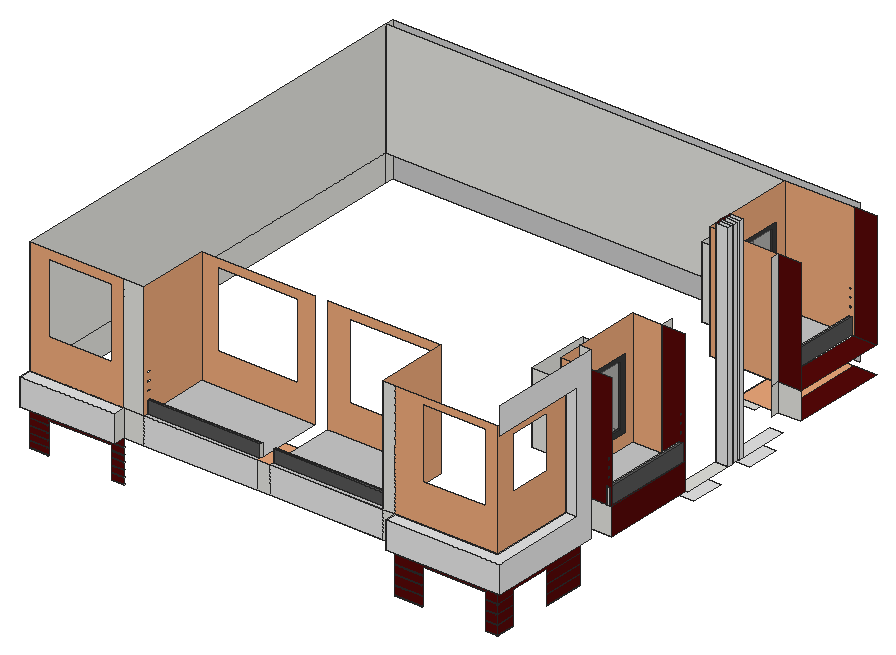
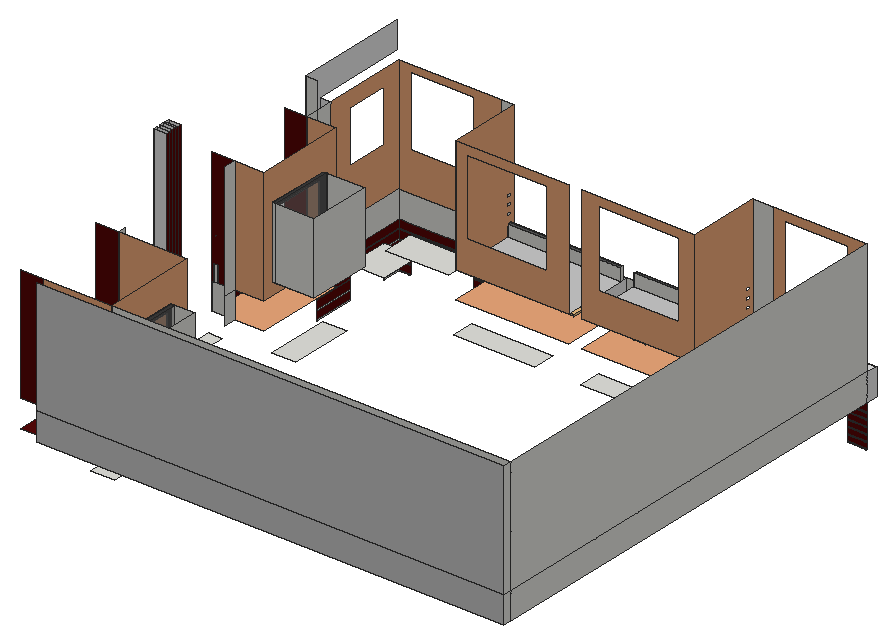
# SketchUp Ruby script. Lengths in inches.
U = 1.inch
M = Sketchup.active_model
def pt(a) = Geom::Point3d.new(a.map { |v| v * U })
def face(e, loops, mat)
  f = e.add_face(loops[0].map { |a| pt(a) })
  loops[1..].each { |l| e.add_face(l.map { |a| pt(a) }).erase! }
  f.material = f.back_material = mat if mat
  f
end
# faces: each face lists its corners as indices into pts; further lists are holes
def faces(e, pts, list, mat = nil) = list.each { |f| face(e, (f[0].is_a?(Array) ? f : [f]).map { |l| l.map { |i| pts[i] } }, mat) }
# xy, xz, yz: faces in a plane at the given z, y or x. An outline is a flat list of corners, or four numbers for a rectangle; further outlines are holes
def ring(l) = l.size == 4 ? [[l[0], l[1]], [l[2], l[1]], [l[2], l[3]], [l[0], l[3]]] : l.each_slice(2).to_a
def flat(e, list, mat, &to3) = list.each { |f| face(e, (f[0].is_a?(Array) ? f : [f]).map { |l| ring(l).map { |u, v| to3.(u, v) } }, mat) }
def xy(e, z, list, mat = nil) = flat(e, list, mat) { |x, y| [x, y, z] }
def xz(e, y, list, mat = nil) = flat(e, list, mat) { |x, z| [x, y, z] }
def yz(e, x, list, mat = nil) = flat(e, list, mat) { |y, z| [x, y, z] }
def lines(e, pts, list) = list.each { |a, b| e.add_line(pt(pts[a]), pt(pts[b])) }
# prism: a flat outline (further loops are holes) pulled along v
def prism(e, loops, v, mat = nil)
  f = face(e, loops, mat); d = Geom::Vector3d.new(v.map { |x| x * U })
  f.pushpull(f.normal.samedirection?(d) ? d.length : -d.length)
end
def box(e, o, s, mat = nil) = prism(e, [[o, [o[0] + s[0], o[1], o[2]], [o[0] + s[0], o[1] + s[1], o[2]], [o[0], o[1] + s[1], o[2]]]], [0, 0, s[2]], mat)
def at(x, y, z, deg = 0) = Geom::Transformation.translation(pt([x, y, z])) * Geom::Transformation.rotation(ORIGIN, Z_AXIS, deg.degrees)
def axes(o, x, y, z) = Geom::Transformation.new([*x, 0, *y, 0, *z, 0, *pt(o).to_a, 1])
def part(name) = M.definitions.add(name)
# library, detail: a bought-in or finely detailed component or shape, given as its bounding box
def library(name, o, s) = part(name).tap { |d| box(d.entities, o, s) }
def detail(e, o, s) = box(e.add_group.entities, o, s)
def put(e, d, t, mat = nil) = e.add_instance(d, t).tap { |i| i.material = mat if mat }
def group(e, t, mat = nil) = e.add_group.tap { |g| g.transformation = t; g.material = mat if mat }.entities
root = M.entities
M.materials.add("Generic").color = [86, 8, 8]
M.materials.add("Generic\#1").color = [236, 168, 122]
M.materials.add("Generic\#4").color = [201, 201, 201]
M.materials.add("Generic\#5").color = [230, 230, 230]
M.materials.add("[Color M06]").color = [86, 86, 86]
M.materials.add("[Color M07]").color = [58, 58, 58]
M.materials.add("[Translucent Glass Gray]").color = [127, 127, 127]
M.materials["[Translucent Glass Gray]"].alpha = 0.35
c1 = library("Tlon Light 450 Ceiling 152 006",[-8.86,-8.86,-3.78],[17.72,17.72,3.56])
c2 = part("Group\#5")
xy(c2.entities,0,[[0,0,6,92.0625]],"[Color M07]")
xy(c2.entities,6.58,[[3,6.58,6,85.48]],"[Color M07]")
xy(c2.entities,96.73,[[3,6.58,6,85.48]],"[Color M07]")
xy(c2.entities,103.3125,[[0,0,6,92.0625]],"[Color M07]")
xz(c2.entities,0,[[0,0,6,103.3125]],"[Color M07]")
xz(c2.entities,6.58,[[3,6.58,6,96.73]],"[Color M07]")
xz(c2.entities,85.48,[[3,6.58,6,96.73]],"[Color M07]")
xz(c2.entities,92.0625,[[0,0,6,103.3125]],"[Color M07]")
yz(c2.entities,0,[[0,0,92.0625,103.3125]],"[Translucent Glass Gray]")
yz(c2.entities,3,[[6.58,6.58,85.48,96.73]],"[Translucent Glass Gray]")
yz(c2.entities,6,[[[0,0,92.0625,103.3125],[6.58,6.58,85.48,96.73]]],"[Color M07]")
xy(root,308.0625,[[549.5625,113.625,589.83,113.625,589.83,113.93,549.5625,113.92],[681.51,113.625,698.4375,113.625,698.4375,113.92,698.14,113.92,681.51,113.93],[698.14,113.92,698.4375,141.33],[698.14,204.02,698.4375,263.625]])
xy(root,309.0625,[[549.5625,113.625,549.5625,113.92,589.83,113.93,589.83,113.625],[681.51,113.625,681.51,113.93,698.14,113.92,698.4375,113.92,698.4375,113.625],[698.14,113.92,698.4375,141.33],[698.14,204.02,698.4375,263.625]])
xy(root,313.875,[[16.6875,113.625,44.83,113.92],[136.51,113.625,154.5,113.92]])
xy(root,314.875,[[16.6875,113.625,44.83,113.92],[136.51,113.625,154.5,113.92]])
xy(root,321.625,[[549.5625,113.625,589.83,113.625,589.83,113.93,549.5625,113.92],[681.51,113.625,698.4375,113.625,698.4375,113.92,698.14,113.92,681.51,113.93],[698.14,113.92,698.4375,141.33],[698.14,204.02,698.4375,263.625]])
xy(root,322.625,[[549.5625,113.625,589.83,113.92],[681.51,113.625,698.4375,113.92],[698.14,113.92,698.4375,141.33],[698.14,204.02,698.4375,263.625]])
xy(root,323.5625,[[16.6875,113.625,44.83,113.92],[136.51,113.625,154.5,113.92]])
xy(root,324.5625,[[16.6875,113.625,44.83,113.92],[136.51,113.625,154.5,113.92]])
xy(root,333.25,[[16.6875,113.625,44.83,113.92],[136.51,113.625,154.5,113.92]])
xy(root,334.25,[[16.6875,113.625,44.83,113.92],[136.51,113.625,154.5,113.92]])
xy(root,335.1875,[[549.5625,113.625,589.83,113.625,589.83,113.93,549.5625,113.92],[681.51,113.625,698.4375,113.625,698.4375,113.92,698.14,113.92,681.51,113.93],[698.14,113.92,698.4375,141.33],[698.14,204.02,698.4375,263.625]])
xy(root,336.1875,[[549.5625,113.625,549.5625,113.92,589.83,113.93,589.83,113.625],[681.51,113.625,681.51,113.93,698.14,113.92,698.4375,113.92,698.4375,113.625],[698.14,113.92,698.4375,141.33],[698.14,204.02,698.4375,263.625]])
xy(root,340.79,[[621.0625,306.16,656.0625,398.23]])
xy(root,342.9375,[[16.6875,113.625,44.83,113.625,44.83,113.93,16.6875,113.92],[136.51,113.625,154.5,113.625,154.5,113.92,136.51,113.93]])
xy(root,343.74,[[686.125,448.93,717.1875,497.24],[686.125,549.8,717.1875,598.12]],"Generic\#5")
xy(root,343.9375,[[16.6875,113.625,16.6875,113.92,44.83,113.93,44.83,113.625],[136.51,113.625,136.51,113.93,154.5,113.92,154.5,113.625]])
xy(root,344.94,[[606.125,655.17,641.125,747.23]])
xy(root,348.75,[[549.5625,113.625,589.83,113.625,589.83,113.93,549.5625,113.92],[681.51,113.625,698.4375,113.625,698.4375,113.92,698.14,113.92,681.51,113.93],[698.14,113.92,698.4375,141.33],[698.14,204.02,698.4375,263.625]])
xy(root,349.75,[[549.5625,113.625,549.5625,113.92,589.83,113.93,589.83,113.625],[681.51,113.625,681.51,113.93,698.14,113.92,698.4375,113.92,698.4375,113.625],[698.14,113.92,698.4375,141.33],[698.14,204.02,698.4375,263.625]])
xy(root,351.52,[[205.67,219.4375,323.42,251.5625],[390.3,219.4375,508.05,251.5625]])
xy(root,352.625,[[16.6875,113.625,44.83,113.625,44.83,113.93,16.6875,113.92],[136.51,113.625,154.5,113.625,154.5,113.92,136.51,113.93]])
xy(root,353.625,[[16.6875,113.625,16.6875,113.92,44.83,113.93,44.83,113.625],[136.51,113.625,136.51,113.93,154.5,113.92,154.5,113.625]])
xy(root,356.11,[[648.625,141.33,698.4375,204.02]])
xy(root,359.68,[[44.83,113.625,136.51,130.0625]])
xy(root,360.11,[[589.83,113.625,681.51,159.375]])
xy(root,361.33,[[698.4375,436.65,717.1875,510.93],[698.4375,510.93,717.1875,516.93],[698.4375,521.18,717.1875,527.18],[698.4375,531.45,717.1875,537.45]])
xy(root,361.33,[[698.4375,516.93,717.1875,521.18],[698.4375,527.18,717.1875,531.45],[698.4375,537.45,717.1875,610.59]],"Generic\#5")
xy(root,362.3125,[[16.6875,113.625,154.5,113.92],[549.5625,113.625,698.4375,113.92],[698.14,113.92,698.4375,263.625]])
xy(root,363.3125,[[16.6875,113.625,154.5,113.92],[549.5625,113.625,698.4375,113.92],[698.14,113.92,698.4375,263.625]])
xy(root,375.3125,[[698.4375,624.8125,731.4375,762.8125]],"Generic")
xy(root,375.3125,[[183.5625,113.625,347.9375,219.4375],[367.1875,113.625,531.5625,219.4375],[656.0625,281.625,731.4375,413.625],[641.125,624.8125,698.4375,762.8125]],"Generic\#1")
xy(root,375.3125,[[16.6875,96.5625,154.5,113.625],[549.5625,96.5625,549.5625,113.625,698.4375,113.625,698.4375,263.625,715.125,263.625,715.125,96.5625]],"Generic\#5")
xy(root,414.625,[[183.5625,119.625,347.9375,123.625],[367.1875,119.625,531.5625,123.625],[723.5625,281.625,728.4375,413.625],[691.5625,624.8125,696.0625,762.8125],[696.0625,624.8125,698.4375,762.8125]])
xy(root,414.625,[[728.4375,281.625,731.4375,413.625],[698.4375,624.8125,731.4375,762.8125]],"Generic")
xy(root,414.625,[[183.5625,113.625,347.9375,119.625],[367.1875,113.625,531.5625,119.625],[183.5625,123.625,347.9375,219.4375],[367.1875,123.625,531.5625,219.4375],[656.0625,281.625,723.5625,413.625],
  [598.75,624.8125,691.5625,762.8125]],"Generic\#4")
xy(root,414.625,[[16.6875,96.5625,154.5,113.625],[549.5625,96.5625,715.125,96.5625,715.125,238.3125,698.4375,238.3125,698.4375,113.625,549.5625,113.625]],"Generic\#5")
xy(root,432.625,[[183.5625,119.625,347.9375,123.625],[367.1875,119.625,531.5625,123.625]],"[Color M06]")
xy(root,433.67,[[594.5625,306.16,656.0625,398.23]])
xy(root,433.84,[[563.75,654.65,598.75,746.71]])
xy(root,438.625,[[723.5625,281.625,728.4375,413.625],[691.5625,624.8125,696.0625,762.8125]],"[Color M06]")
xz(root,96.5625,[[16.6875,375.3125,154.5,414.625],[549.5625,375.3125,715.125,414.625]],"Generic\#5")
xz(root,113.625,[[16.6875,375.3125,154.5,413],[154.5,375.3125,183.4375,414.625],[347.9375,375.3125,367.1875,414.625],[531.6875,375.3125,549.5625,414.625],[549.5625,375.3125,698.4375,414.625],
  [16.6875,413,154.5,414],[16.6875,414,154.5,414.625],[154.5,414.625,183.4375,582.625],[183.4375,414.625,183.5625,582.625],[531.5625,414.625,531.6875,582.625],
  [531.6875,414.625,549.5625,582.625]])
xz(root,113.625,[[549.5625,309.0625,589.83,321.625],[681.51,309.0625,698.4375,321.625],[16.6875,314.875,44.83,323.5625],[136.51,314.875,154.5,323.5625],[549.5625,322.625,589.83,335.1875],
  [681.51,322.625,698.4375,335.1875],[16.6875,324.5625,44.83,333.25],[136.51,324.5625,154.5,333.25],[16.6875,334.25,44.83,342.9375],[136.51,334.25,154.5,342.9375],
  [549.5625,336.1875,589.83,348.75],[681.51,336.1875,698.4375,348.75],[16.6875,343.9375,44.83,352.625],[136.51,343.9375,154.5,352.625],[549.5625,349.75,589.83,349.75,589.83,360.11,681.51,360.11,681.51,349.75,698.4375,349.75,698.4375,362.3125,549.5625,362.3125],
  [16.6875,353.625,44.83,353.625,44.83,359.68,136.51,359.68,136.51,353.625,154.5,353.625,154.5,362.3125,16.6875,362.3125],[16.6875,363.3125,154.5,375.3125],[549.5625,363.3125,698.4375,375.3125]],"Generic")
xz(root,113.625,[[[16.6875,414.625,154.5,582.625],[44.83,468.8,136.51,570.24]],[[549.5625,414.625,698.4375,582.625],[589.83,471.43,681.51,572.86]]],"Generic\#1")
xz(root,113.625,[[183.4375,375.3125,347.9375,414.625],[367.1875,375.3125,531.6875,414.625]],"Generic\#5")
xz(root,113.92,[[16.6875,313.875,44.83,314.875],[136.51,313.875,154.5,314.875],[16.6875,323.5625,44.83,324.5625],[136.51,323.5625,154.5,324.5625],[16.6875,333.25,44.83,334.25],
  [136.51,333.25,154.5,334.25],[16.6875,362.3125,154.5,363.3125],[549.5625,362.3125,698.14,363.3125]])
xz(root,119.625,[[183.5625,414.625,347.9375,432.625],[367.1875,414.625,531.5625,432.625]],"[Color M06]")
xz(root,123.625,[[183.5625,414.625,347.9375,432.625],[367.1875,414.625,531.5625,432.625]])
xz(root,141.33,[[698.14,308.0625,698.4375,309.0625],[698.14,321.625,698.4375,322.625],[698.14,335.1875,698.4375,336.1875],[698.14,348.75,698.4375,349.75]])
xz(root,204.02,[[698.14,308.0625,698.4375,309.0625],[698.14,321.625,698.4375,322.625],[698.14,335.1875,698.4375,336.1875],[698.14,348.75,698.4375,349.75]])
xz(root,219.4375,[[[183.5625,414.625,347.9375,582.625],[205.67,460.21,323.42,570.34]],[[367.1875,414.625,531.5625,582.625],[397.99,460.21,515.74,570.34]]],"Generic\#1")
xz(root,238.3125,[[698.4375,414.625,715.125,582.625]],"Generic\#5")
xz(root,263.625,[[698.14,308.0625,698.4375,309.0625],[698.14,321.625,698.4375,322.625],[698.14,335.1875,698.4375,336.1875],[698.14,348.75,698.4375,349.75],[698.14,362.3125,698.4375,363.3125],
  [698.4375,375.3125,715.125,414.625],[698.4375,414.625,715.125,621.9375]])
xz(root,281.625,[[698.4375,375.3125,731.4375,414.625],[723.5625,414.625,728.4375,438.625]])
xz(root,281.625,[[[698.4375,414.625,698.4375,582.625,731.4375,582.625,731.4375,414.625,728.4375,414.625,728.4375,438.625,723.5625,438.625,723.5625,414.625],[724.45,473.55,727.82,476.68],[724.45,461.67,727.82,464.79],[724.45,449.67,727.82,452.79]]],"Generic")
xz(root,281.625,[[656.0625,414.625,698.4375,582.625]],"Generic\#1")
xz(root,306.16,[[594.5625,433.67,656.0625,536.98]])
xz(root,398.23,[[594.5625,433.67,656.0625,536.98]])
xz(root,413.625,[[698.4375,375.3125,731.4375,414.625],[723.5625,414.625,728.4375,438.625]])
xz(root,413.625,[[[698.4375,414.625,723.5625,414.625,723.5625,438.625,728.4375,438.625,728.4375,414.625,731.4375,414.625,731.4375,582.625,698.4375,582.625],[724.45,449.67,727.82,452.79],[724.45,461.67,727.82,464.79],[724.45,473.55,727.82,476.68]]],"Generic")
xz(root,413.625,[[656.0625,414.625,698.4375,582.625]],"Generic\#1")
xz(root,510.93,[[698.4375,361.33,717.1875,672.98]],"Generic\#5")
xz(root,516.93,[[698.4375,361.33,717.1875,672.98]],"Generic\#5")
xz(root,521.18,[[698.4375,361.33,717.1875,672.98]],"Generic\#5")
xz(root,527.18,[[698.4375,361.33,717.1875,672.98]],"Generic\#5")
xz(root,531.45,[[698.4375,361.33,717.1875,672.98]],"Generic\#5")
xz(root,537.45,[[698.4375,361.33,717.1875,672.98]],"Generic\#5")
xz(root,624.8125,[[698.4375,375.3125,731.4375,414.625],[691.5625,414.625,696.0625,438.625]])
xz(root,624.8125,[[698.4375,414.625,731.4375,582.625]],"Generic")
xz(root,624.8125,[[[598.75,414.625,598.75,582.625,698.4375,582.625,698.4375,414.625,696.0625,414.625,696.0625,438.625,691.5625,438.625,691.5625,414.625],[691.43,473.54,695.61,476.85],[691.43,461.54,695.61,464.85],[691.43,449.49,695.61,452.8]]],"Generic\#1")
xz(root,654.65,[[563.75,433.84,598.75,537.15]])
xz(root,746.71,[[563.75,433.84,598.75,537.15]])
xz(root,762.8125,[[16.6875,414.625,598.75,582.625],[691.5625,414.625,696.0625,438.625]])
xz(root,762.8125,[[698.4375,414.625,731.4375,582.625]],"Generic")
xz(root,762.8125,[[[598.75,414.625,691.5625,414.625,691.5625,438.625,696.0625,438.625,696.0625,414.625,698.4375,414.625,698.4375,582.625,598.75,582.625],[691.43,449.49,695.61,452.8],[691.43,461.54,695.61,464.85],[691.43,473.54,695.61,476.85]]],"Generic\#1")
xz(root,774.8125,[[16.6875,375.3125,698.4375,414.625],[16.6875,414.625,698.4375,582.625]],"Generic\#4")
yz(root,16.6875,[[113.625,375.3125,762.8125,414.625],[762.8125,375.3125,774.8125,414.625],[113.625,414.625,762.8125,582.625],[762.8125,414.625,774.8125,582.625]])
yz(root,16.6875,[[96.5625,375.3125,113.625,414.625]],"Generic\#5")
yz(root,154.5,[[113.625,313.875,113.92,314.875],[113.625,323.5625,113.92,324.5625],[113.625,333.25,113.92,334.25],[113.625,342.9375,113.92,343.9375],[113.625,352.625,113.92,353.625],
  [113.625,362.3125,113.92,363.3125],[96.5625,375.3125,113.625,414.625]])
yz(root,183.5625,[[119.625,414.625,123.625,432.625]])
yz(root,183.5625,[[[113.625,414.625,119.625,414.625,119.625,432.625,123.625,432.625,123.625,414.625,219.4375,414.625,219.4375,582.625,113.625,582.625],[118.5,466.73,125.9375,470.54],[118.5,454.38,125.9375,458.19],[118.5,442.38,125.9375,446.19]]],"Generic\#1")
yz(root,347.9375,[[119.625,414.625,123.625,432.625]])
yz(root,367.1875,[[119.625,414.625,123.625,432.625]])
yz(root,531.5625,[[119.625,414.625,123.625,432.625]])
yz(root,531.5625,[[[113.625,414.625,113.625,582.625,219.4375,582.625,219.4375,414.625,123.625,414.625,123.625,432.625,119.625,432.625,119.625,414.625],[118.5,466.82,125.9375,470.63],[118.5,454.82,125.9375,458.63],[118.5,442.82,125.9375,446.63]]],"Generic\#1")
yz(root,549.5625,[[113.625,308.0625,113.92,309.0625],[113.625,321.625,113.92,322.625],[113.625,335.1875,113.92,336.1875],[113.625,348.75,113.92,349.75],[113.625,362.3125,113.92,363.3125],
  [96.5625,375.3125,113.625,414.625]])
yz(root,563.75,[[654.65,433.84,746.71,537.15]])
yz(root,594.5625,[[306.16,433.67,398.23,536.98]])
yz(root,598.75,[[[624.8125,414.625,762.8125,582.625],[654.65,433.84,746.71,537.15]]],"Generic\#1")
yz(root,656.0625,[[[281.625,414.625,413.625,582.625],[306.16,433.67,398.23,536.98]]],"Generic\#1")
yz(root,691.5625,[[624.8125,414.625,762.8125,438.625]])
yz(root,696.0625,[[624.8125,414.625,762.8125,438.625]],"[Color M06]")
yz(root,698.14,[[113.92,308.0625,141.33,309.0625],[204.02,308.0625,263.625,309.0625],[113.92,321.625,141.33,322.625],[204.02,321.625,263.625,322.625],[113.92,335.1875,141.33,336.1875],
  [204.02,335.1875,263.625,336.1875],[113.92,348.75,141.33,349.75],[204.02,348.75,263.625,349.75],[113.92,362.3125,263.625,363.3125]])
yz(root,698.4375,[[113.625,375.3125,263.625,414.625],[263.625,375.3125,281.625,414.625],[413.625,375.3125,431.625,414.625],[612.8125,375.3125,624.8125,414.625],[238.3125,414.625,263.625,582.625],
  [263.625,414.625,281.625,582.625],[413.625,414.625,431.625,582.625],[612.8125,414.625,624.8125,582.625]])
yz(root,698.4375,[[113.625,309.0625,141.33,321.625],[204.02,309.0625,263.625,321.625],[113.625,322.625,141.33,335.1875],[204.02,322.625,263.625,335.1875],[113.625,336.1875,141.33,348.75],
  [204.02,336.1875,263.625,348.75],[113.625,349.75,141.33,349.75,141.33,356.11,204.02,356.11,204.02,349.75,263.625,349.75,263.625,362.3125,113.625,362.3125],[510.93,361.33,516.93,672.98],[516.93,361.33,521.18,672.98],[521.18,361.33,527.18,672.98],
  [527.18,361.33,531.45,672.98],[531.45,361.33,537.45,672.98],[113.625,363.3125,263.625,375.3125]],"Generic")
yz(root,698.4375,[[[113.625,414.625,238.3125,582.625],[141.33,483.99,204.02,559.61]]],"Generic\#1")
yz(root,715.125,[[96.5625,375.3125,263.625,375.3125,263.625,621.9375,96.5625,621.9375,96.5625,582.625,238.3125,582.625,238.3125,414.625,96.5625,414.625]],"Generic\#5")
yz(root,717.1875,[[510.93,361.33,516.93,672.98],[521.18,361.33,527.18,672.98],[531.45,361.33,537.45,672.98]],"Generic\#5")
yz(root,723.5625,[[281.625,414.625,413.625,438.625]])
yz(root,728.4375,[[281.625,414.625,413.625,438.625]],"[Color M06]")
yz(root,731.4375,[[281.625,375.3125,413.625,414.625]],"Generic")
p = [[549.5625,113.92,308.0625],[589.83,113.93,308.0625],[589.83,113.93,309.0625],[549.5625,113.92,309.0625],[681.51,113.93,308.0625],[698.14,113.92,308.0625],
  [698.14,113.92,309.0625],[681.51,113.93,309.0625],[549.5625,113.92,321.625],[589.83,113.93,321.625],[589.83,113.92,322.625],[549.5625,113.92,322.625],
  [681.51,113.93,321.625],[698.14,113.92,321.625],[698.14,113.92,322.625],[681.51,113.92,322.625],[549.5625,113.92,335.1875],[589.83,113.93,335.1875],
  [589.83,113.93,336.1875],[549.5625,113.92,336.1875],[681.51,113.93,335.1875],[698.14,113.92,335.1875],[698.14,113.92,336.1875],[681.51,113.93,336.1875],
  [16.6875,113.92,342.9375],[44.83,113.93,342.9375],[44.83,113.93,343.9375],[16.6875,113.92,343.9375],[154.5,113.92,342.9375],[154.5,113.92,343.9375],
  [136.51,113.93,343.9375],[136.51,113.93,342.9375],[549.5625,113.92,348.75],[589.83,113.93,348.75],[589.83,113.93,349.75],[549.5625,113.92,349.75],
  [681.51,113.93,348.75],[698.14,113.92,348.75],[698.14,113.92,349.75],[681.51,113.93,349.75],[16.6875,113.92,352.625],[44.83,113.93,352.625],
  [44.83,113.93,353.625],[16.6875,113.92,353.625],[154.5,113.92,352.625],[154.5,113.92,353.625],[136.51,113.93,353.625],[136.51,113.93,352.625]]
faces(root,p,[[0,1,2,3],[4,5,6,7],[8,9,10,11],[12,13,14,15],[16,17,18,19],[20,21,22,23],[24,25,26,27],[28,29,30,31],
  [32,33,34,35],[36,37,38,39],[40,41,42,43],[44,45,46,47]])
put(root,c1,at(494.27,156.14,377.35))
put(root,c1,at(411.33,156.14,377.35))
put(root,c1,at(306.77,156.14,377.35))
put(root,c1,at(221.27,156.14,377.35))
put(root,c2,at(650.0625,306.16,433.67))
put(root,c2,at(592.75,654.65,433.84))
